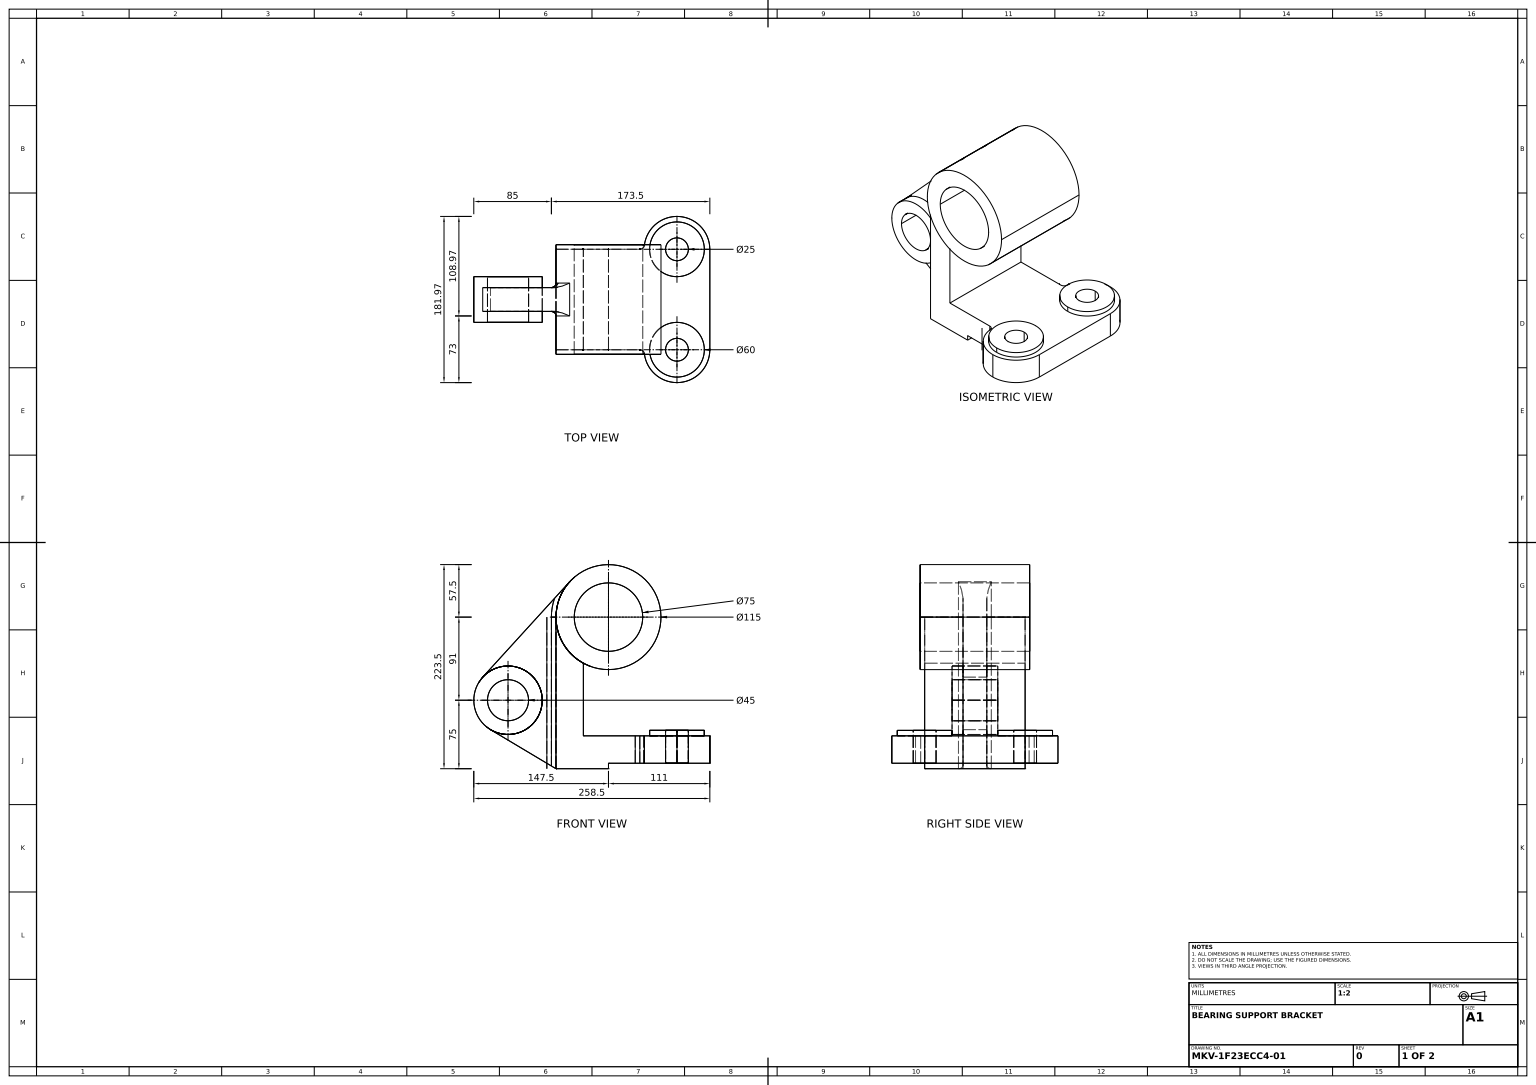
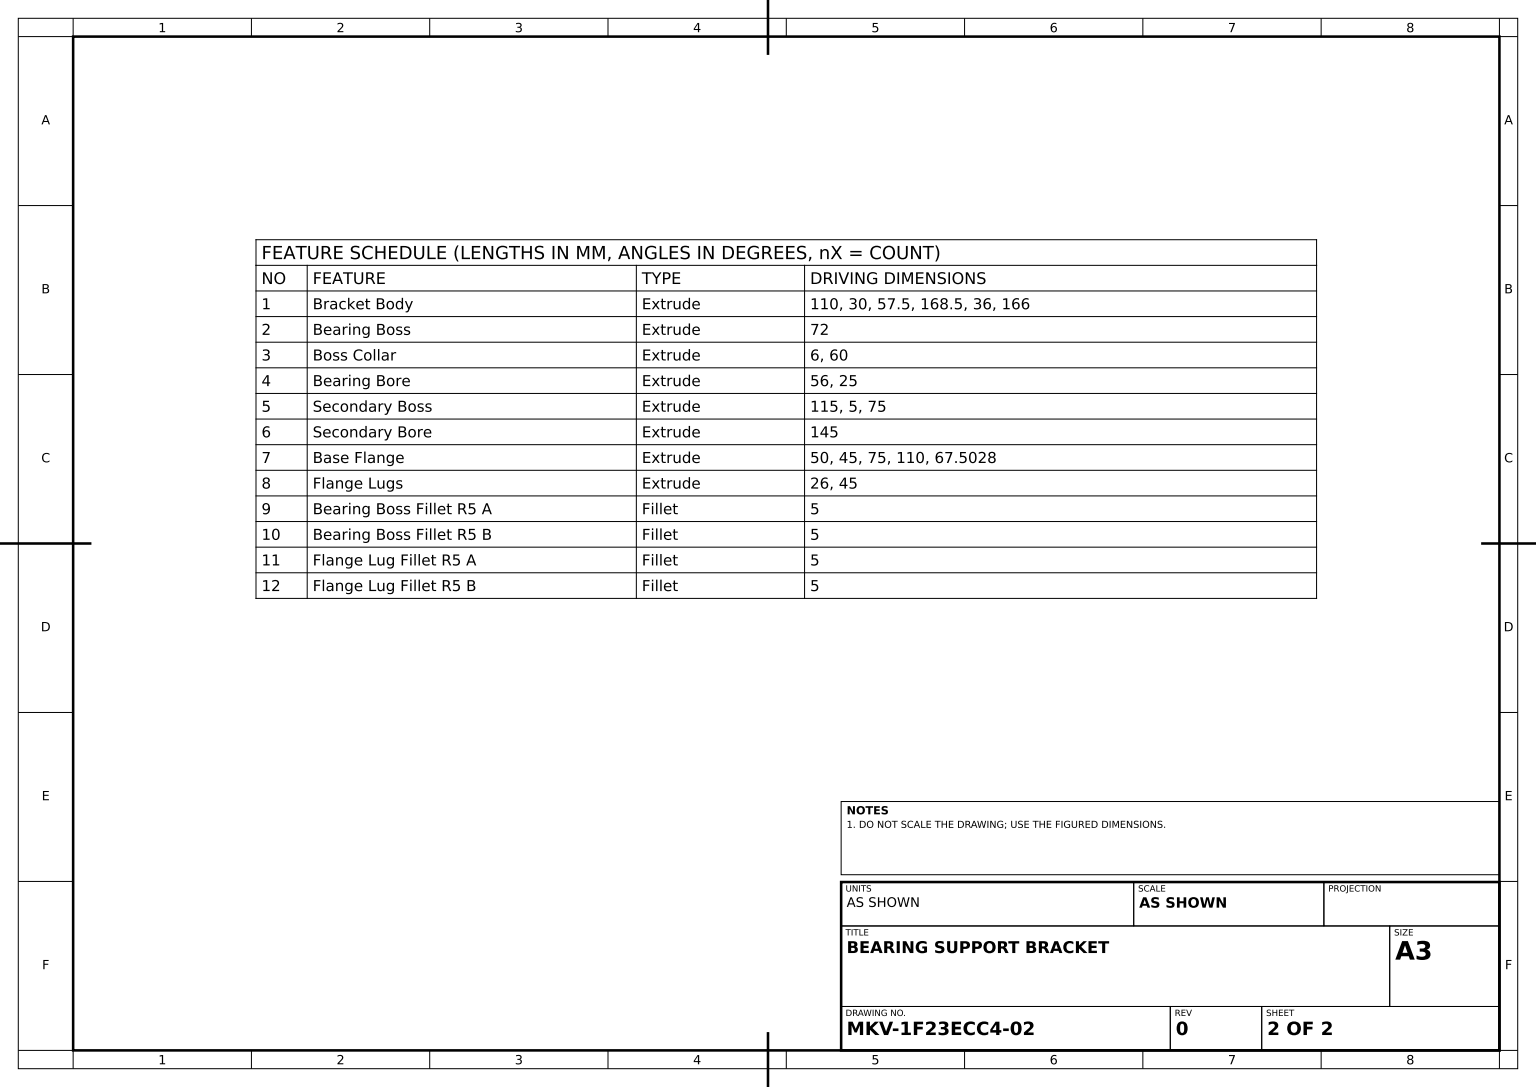
ISO-10303-21;
HEADER;
FILE_DESCRIPTION((''),'2;1');
FILE_NAME('','',(''),(''),'','','');
FILE_SCHEMA(('AUTOMOTIVE_DESIGN'));
ENDSEC;
DATA;
#1=APPLICATION_CONTEXT('');
#2=PRODUCT_CONTEXT('',#1,'mechanical');
#3=PRODUCT('','','',(#2));
#4=PRODUCT_DEFINITION_FORMATION('','',#3);
#5=PRODUCT_DEFINITION_CONTEXT('',#1,'design');
#6=PRODUCT_DEFINITION('','',#4,#5);
#7=PRODUCT_DEFINITION_SHAPE('','',#6);
#8=(LENGTH_UNIT()NAMED_UNIT(*)SI_UNIT(.MILLI.,.METRE.));
#9=(NAMED_UNIT(*)PLANE_ANGLE_UNIT()SI_UNIT($,.RADIAN.));
#10=(NAMED_UNIT(*)SI_UNIT($,.STERADIAN.)SOLID_ANGLE_UNIT());
#11=UNCERTAINTY_MEASURE_WITH_UNIT(LENGTH_MEASURE(1.E-05),#8,'distance_accuracy_value','');
#12=(GEOMETRIC_REPRESENTATION_CONTEXT(3)GLOBAL_UNCERTAINTY_ASSIGNED_CONTEXT((#11))GLOBAL_UNIT_ASSIGNED_CONTEXT((#8,#9,#10))REPRESENTATION_CONTEXT('',''));
#13=CARTESIAN_POINT('',(-75.,75.,-25.));
#14=VERTEX_POINT('',#13);
#15=CARTESIAN_POINT('',(-30.,75.,-25.));
#16=VERTEX_POINT('',#15);
#17=CARTESIAN_POINT('',(-52.5,75.,-25.));
#18=DIRECTION('',(0.,0.,1.));
#19=DIRECTION('',(1.,0.,0.));
#20=AXIS2_PLACEMENT_3D('',#17,#18,#19);
#21=CIRCLE('',#20,22.5);
#22=EDGE_CURVE('',#14,#16,#21,.T.);
#23=ORIENTED_EDGE('',*,*,#22,.T.);
#24=EDGE_CURVE('',#16,#14,#21,.T.);
#25=ORIENTED_EDGE('',*,*,#24,.T.);
#26=EDGE_LOOP('',(#23,#25));
#27=FACE_BOUND('',#26,.T.);
#28=CARTESIAN_POINT('',(-15.,75.,-25.));
#29=VERTEX_POINT('',#28);
#30=CARTESIAN_POINT('',(-90.,75.,-25.));
#31=VERTEX_POINT('',#30);
#32=CIRCLE('',#20,37.5);
#33=EDGE_CURVE('',#29,#31,#32,.T.);
#34=ORIENTED_EDGE('',*,*,#33,.F.);
#35=EDGE_CURVE('',#31,#29,#32,.T.);
#36=ORIENTED_EDGE('',*,*,#35,.F.);
#37=EDGE_LOOP('',(#34,#36));
#38=FACE_OUTER_BOUND('',#37,.T.);
#39=CARTESIAN_POINT('',(0.,0.,-25.));
#40=AXIS2_PLACEMENT_3D('',#39,#18,#19);
#41=PLANE('',#40);
#42=ADVANCED_FACE('',(#27,#38),#41,.F.);
#43=CARTESIAN_POINT('',(30.,36.,55.));
#44=VERTEX_POINT('',#43);
#45=CARTESIAN_POINT('',(30.,115.502475,55.));
#46=VERTEX_POINT('',#45);
#47=DIRECTION('',(0.,1.,0.));
#48=VECTOR('',#47,1000.);
#49=LINE('',#43,#48);
#50=EDGE_CURVE('',#44,#46,#49,.T.);
#51=ORIENTED_EDGE('',*,*,#50,.F.);
#52=CARTESIAN_POINT('',(30.,36.,-55.));
#53=VERTEX_POINT('',#52);
#54=DIRECTION('',(0.,0.,-1.));
#55=VECTOR('',#54,1000.);
#56=LINE('',#43,#55);
#57=EDGE_CURVE('',#44,#53,#56,.T.);
#58=ORIENTED_EDGE('',*,*,#57,.T.);
#59=CARTESIAN_POINT('',(30.,115.502475,-55.));
#60=VERTEX_POINT('',#59);
#61=LINE('',#52,#48);
#62=EDGE_CURVE('',#53,#60,#61,.T.);
#63=ORIENTED_EDGE('',*,*,#62,.T.);
#64=CARTESIAN_POINT('',(30.,115.502475,60.));
#65=LINE('',#64,#55);
#66=EDGE_CURVE('',#46,#60,#65,.T.);
#67=ORIENTED_EDGE('',*,*,#66,.F.);
#68=EDGE_LOOP('',(#51,#58,#63,#67));
#69=FACE_OUTER_BOUND('',#68,.T.);
#70=DIRECTION('',(-1.,0.,0.));
#71=DIRECTION('',(0.,-1.,0.));
#72=AXIS2_PLACEMENT_3D('',#43,#70,#71);
#73=PLANE('',#72);
#74=ADVANCED_FACE('',(#69),#73,.F.);
#75=CARTESIAN_POINT('',(-1.497355,186.629157,13.));
#76=VERTEX_POINT('',#75);
#77=CARTESIAN_POINT('',(-80.215573,100.260582,13.));
#78=VERTEX_POINT('',#77);
#79=DIRECTION('',(-0.673615532,-0.73908194,0.));
#80=VECTOR('',#79,1000.);
#81=LINE('',#77,#80);
#82=EDGE_CURVE('',#76,#78,#81,.T.);
#83=ORIENTED_EDGE('',*,*,#82,.F.);
#84=CARTESIAN_POINT('',(15.002788,204.732893,18.));
#85=VERTEX_POINT('',#84);
#86=CARTESIAN_POINT('',(-0.790057,187.405195,13.));
#87=CARTESIAN_POINT('',(-0.086672,188.176939,13.050128));
#88=CARTESIAN_POINT('',(1.314429,189.714209,13.222969));
#89=CARTESIAN_POINT('',(2.012125,190.479711,13.345952));
#90=CARTESIAN_POINT('',(4.098718,192.769093,13.798084));
#91=CARTESIAN_POINT('',(5.483281,194.288217,14.210374));
#92=CARTESIAN_POINT('',(8.22755,197.299192,15.156454));
#93=CARTESIAN_POINT('',(9.588678,198.792603,15.691176));
#94=CARTESIAN_POINT('',(11.622818,201.024434,16.535584));
#95=CARTESIAN_POINT('',(12.299582,201.766971,16.824242));
#96=CARTESIAN_POINT('',(13.313784,202.87974,17.262515));
#97=CARTESIAN_POINT('',(13.651694,203.250491,17.40949));
#98=CARTESIAN_POINT('',(14.327357,203.991818,17.704321));
#99=CARTESIAN_POINT('',(14.665836,204.363193,17.852495));
#100=B_SPLINE_CURVE_WITH_KNOTS('',3,(#75,#86,#87,#88,#89,#90,#91,#92,#93,#94,#95,#96,#97,#98,#99,#84),.UNSPECIFIED.,.F.,.F.,(4,2,2,2,2,2,2,4),(0.,0.003129059,0.006258119,0.012516238,0.018774357,0.021903416,0.023467946,0.025032475),.UNSPECIFIED.);
#101=EDGE_CURVE('',#76,#85,#100,.T.);
#102=ORIENTED_EDGE('',*,*,#101,.T.);
#103=CARTESIAN_POINT('',(15.002788,204.732893,-18.));
#104=VERTEX_POINT('',#103);
#105=CARTESIAN_POINT('',(15.002788,204.732893,13.));
#106=LINE('',#105,#55);
#107=EDGE_CURVE('',#85,#104,#106,.T.);
#108=ORIENTED_EDGE('',*,*,#107,.T.);
#109=CARTESIAN_POINT('',(-1.497355,186.629157,-13.));
#110=VERTEX_POINT('',#109);
#111=CARTESIAN_POINT('',(13.652305,203.251161,-17.408809));
#112=CARTESIAN_POINT('',(12.300813,201.768322,-16.817032));
#113=CARTESIAN_POINT('',(9.588636,198.792558,-15.69116));
#114=CARTESIAN_POINT('',(8.227513,197.299152,-15.15644));
#115=CARTESIAN_POINT('',(5.483255,194.288189,-14.210366));
#116=CARTESIAN_POINT('',(4.098697,192.76907,-13.798079));
#117=CARTESIAN_POINT('',(2.012112,190.479697,-13.345949));
#118=CARTESIAN_POINT('',(1.314419,189.714197,-13.222967));
#119=CARTESIAN_POINT('',(-0.086678,188.176933,-13.050128));
#120=CARTESIAN_POINT('',(-0.790059,187.405192,-13.));
#121=B_SPLINE_CURVE_WITH_KNOTS('',3,(#103,#111,#112,#113,#114,#115,#116,#117,#118,#119,#120,#109),.UNSPECIFIED.,.F.,.F.,(4,2,2,2,2,4),(-0.000047958,0.006222574,0.012493106,0.018763638,0.021898904,0.025034171),.UNSPECIFIED.);
#122=EDGE_CURVE('',#104,#110,#121,.T.);
#123=ORIENTED_EDGE('',*,*,#122,.T.);
#124=CARTESIAN_POINT('',(-80.215573,100.260582,-13.));
#125=VERTEX_POINT('',#124);
#126=LINE('',#124,#80);
#127=EDGE_CURVE('',#110,#125,#126,.T.);
#128=ORIENTED_EDGE('',*,*,#127,.T.);
#129=LINE('',#77,#55);
#130=EDGE_CURVE('',#78,#125,#129,.T.);
#131=ORIENTED_EDGE('',*,*,#130,.F.);
#132=EDGE_LOOP('',(#83,#102,#108,#123,#128,#131));
#133=FACE_OUTER_BOUND('',#132,.T.);
#134=DIRECTION('',(0.73908194,-0.673615532,0.));
#135=DIRECTION('',(0.673615532,0.73908194,0.));
#136=AXIS2_PLACEMENT_3D('',#77,#134,#135);
#137=PLANE('',#136);
#138=ADVANCED_FACE('',(#133),#137,.F.);
#139=CARTESIAN_POINT('',(-90.,75.,25.));
#140=VERTEX_POINT('',#139);
#141=CARTESIAN_POINT('',(-15.,75.,25.));
#142=VERTEX_POINT('',#141);
#143=CARTESIAN_POINT('',(-52.5,75.,25.));
#144=AXIS2_PLACEMENT_3D('',#143,#18,#19);
#145=CIRCLE('',#144,37.5);
#146=EDGE_CURVE('',#140,#142,#145,.T.);
#147=ORIENTED_EDGE('',*,*,#146,.F.);
#148=CARTESIAN_POINT('',(-90.,75.,13.));
#149=LINE('',#148,#55);
#150=EDGE_CURVE('',#140,#31,#149,.T.);
#151=ORIENTED_EDGE('',*,*,#150,.T.);
#152=ORIENTED_EDGE('',*,*,#35,.T.);
#153=CARTESIAN_POINT('',(-15.,75.,-13.));
#154=VERTEX_POINT('',#153);
#155=CARTESIAN_POINT('',(-15.,75.,13.));
#156=LINE('',#155,#55);
#157=EDGE_CURVE('',#154,#29,#156,.T.);
#158=ORIENTED_EDGE('',*,*,#157,.F.);
#159=CARTESIAN_POINT('',(-71.716935,42.798146,-13.));
#160=VERTEX_POINT('',#159);
#161=CARTESIAN_POINT('',(-52.5,75.,-13.));
#162=AXIS2_PLACEMENT_3D('',#161,#54,#19);
#163=CIRCLE('',#162,37.5);
#164=EDGE_CURVE('',#154,#160,#163,.T.);
#165=ORIENTED_EDGE('',*,*,#164,.T.);
#166=CARTESIAN_POINT('',(-71.716935,42.798146,13.));
#167=VERTEX_POINT('',#166);
#168=LINE('',#166,#55);
#169=EDGE_CURVE('',#167,#160,#168,.T.);
#170=ORIENTED_EDGE('',*,*,#169,.F.);
#171=VERTEX_POINT('',#155);
#172=CARTESIAN_POINT('',(-52.5,75.,13.));
#173=AXIS2_PLACEMENT_3D('',#172,#54,#19);
#174=CIRCLE('',#173,37.5);
#175=EDGE_CURVE('',#171,#167,#174,.T.);
#176=ORIENTED_EDGE('',*,*,#175,.F.);
#177=EDGE_CURVE('',#142,#171,#156,.T.);
#178=ORIENTED_EDGE('',*,*,#177,.F.);
#179=EDGE_LOOP('',(#147,#151,#152,#158,#165,#170,#176,#178));
#180=FACE_OUTER_BOUND('',#179,.T.);
#181=AXIS2_PLACEMENT_3D('',#172,#54,#70);
#182=CYLINDRICAL_SURFACE('',#181,37.5);
#183=ADVANCED_FACE('',(#180),#182,.T.);
#184=CARTESIAN_POINT('',(96.768701,36.,59.390244));
#185=VERTEX_POINT('',#184);
#186=CARTESIAN_POINT('',(96.768701,6.,59.390244));
#187=VERTEX_POINT('',#186);
#188=CARTESIAN_POINT('',(96.768701,-95.823376,59.390244));
#189=VECTOR('',#71,1000.);
#190=LINE('',#188,#189);
#191=EDGE_CURVE('',#185,#187,#190,.T.);
#192=ORIENTED_EDGE('',*,*,#191,.T.);
#193=CARTESIAN_POINT('',(132.5,6.,91.));
#194=VERTEX_POINT('',#193);
#195=CARTESIAN_POINT('',(132.5,6.,55.));
#196=AXIS2_PLACEMENT_3D('',#195,#71,#70);
#197=CIRCLE('',#196,36.);
#198=EDGE_CURVE('',#194,#187,#197,.T.);
#199=ORIENTED_EDGE('',*,*,#198,.F.);
#200=CARTESIAN_POINT('',(132.5,36.,91.));
#201=VERTEX_POINT('',#200);
#202=CARTESIAN_POINT('',(132.5,-95.823376,91.));
#203=LINE('',#202,#48);
#204=EDGE_CURVE('',#194,#201,#203,.T.);
#205=ORIENTED_EDGE('',*,*,#204,.T.);
#206=CARTESIAN_POINT('',(132.5,36.,55.));
#207=AXIS2_PLACEMENT_3D('',#206,#47,#18);
#208=CIRCLE('',#207,36.);
#209=EDGE_CURVE('',#185,#201,#208,.T.);
#210=ORIENTED_EDGE('',*,*,#209,.F.);
#211=EDGE_LOOP('',(#192,#199,#205,#210));
#212=FACE_OUTER_BOUND('',#211,.T.);
#213=CARTESIAN_POINT('',(132.5,-95.823376,55.));
#214=AXIS2_PLACEMENT_3D('',#213,#47,#18);
#215=CYLINDRICAL_SURFACE('',#214,36.);
#216=ADVANCED_FACE('',(#212),#215,.T.);
#217=CARTESIAN_POINT('',(96.768701,6.,-59.390244));
#218=VERTEX_POINT('',#217);
#219=CARTESIAN_POINT('',(96.768701,36.,-59.390244));
#220=VERTEX_POINT('',#219);
#221=CARTESIAN_POINT('',(96.768701,-95.823376,-59.390244));
#222=LINE('',#221,#48);
#223=EDGE_CURVE('',#218,#220,#222,.T.);
#224=ORIENTED_EDGE('',*,*,#223,.T.);
#225=CARTESIAN_POINT('',(168.5,36.,-55.));
#226=VERTEX_POINT('',#225);
#227=CARTESIAN_POINT('',(132.5,36.,-55.));
#228=AXIS2_PLACEMENT_3D('',#227,#47,#18);
#229=CIRCLE('',#228,36.);
#230=EDGE_CURVE('',#226,#220,#229,.T.);
#231=ORIENTED_EDGE('',*,*,#230,.F.);
#232=CARTESIAN_POINT('',(168.5,6.,-55.));
#233=VERTEX_POINT('',#232);
#234=LINE('',#232,#48);
#235=EDGE_CURVE('',#233,#226,#234,.T.);
#236=ORIENTED_EDGE('',*,*,#235,.F.);
#237=CARTESIAN_POINT('',(132.5,6.,-55.));
#238=AXIS2_PLACEMENT_3D('',#237,#71,#70);
#239=CIRCLE('',#238,36.);
#240=EDGE_CURVE('',#218,#233,#239,.T.);
#241=ORIENTED_EDGE('',*,*,#240,.F.);
#242=EDGE_LOOP('',(#224,#231,#236,#241));
#243=FACE_OUTER_BOUND('',#242,.T.);
#244=CARTESIAN_POINT('',(132.5,-95.823376,-55.));
#245=AXIS2_PLACEMENT_3D('',#244,#47,#18);
#246=CYLINDRICAL_SURFACE('',#245,36.);
#247=ADVANCED_FACE('',(#243),#246,.T.);
#248=CARTESIAN_POINT('',(95.,166.,60.));
#249=VERTEX_POINT('',#248);
#250=CARTESIAN_POINT('',(95.,166.,-60.));
#251=VERTEX_POINT('',#250);
#252=LINE('',#248,#55);
#253=EDGE_CURVE('',#249,#251,#252,.T.);
#254=ORIENTED_EDGE('',*,*,#253,.T.);
#255=CARTESIAN_POINT('',(20.,166.,-60.));
#256=VERTEX_POINT('',#255);
#257=CARTESIAN_POINT('',(57.5,166.,-60.));
#258=AXIS2_PLACEMENT_3D('',#257,#18,#19);
#259=CIRCLE('',#258,37.5);
#260=EDGE_CURVE('',#256,#251,#259,.T.);
#261=ORIENTED_EDGE('',*,*,#260,.F.);
#262=CARTESIAN_POINT('',(20.,166.,60.));
#263=VERTEX_POINT('',#262);
#264=LINE('',#262,#55);
#265=EDGE_CURVE('',#263,#256,#264,.T.);
#266=ORIENTED_EDGE('',*,*,#265,.F.);
#267=CARTESIAN_POINT('',(57.5,166.,60.));
#268=AXIS2_PLACEMENT_3D('',#267,#18,#19);
#269=CIRCLE('',#268,37.5);
#270=EDGE_CURVE('',#263,#249,#269,.T.);
#271=ORIENTED_EDGE('',*,*,#270,.T.);
#272=EDGE_LOOP('',(#254,#261,#266,#271));
#273=FACE_OUTER_BOUND('',#272,.T.);
#274=AXIS2_PLACEMENT_3D('',#267,#54,#70);
#275=CYLINDRICAL_SURFACE('',#274,37.5);
#276=ADVANCED_FACE('',(#273),#275,.F.);
#277=CARTESIAN_POINT('',(-5.,166.,-13.));
#278=VERTEX_POINT('',#277);
#279=CARTESIAN_POINT('',(57.5,166.,-13.));
#280=AXIS2_PLACEMENT_3D('',#279,#18,#19);
#281=CIRCLE('',#280,62.5);
#282=EDGE_CURVE('',#110,#278,#281,.T.);
#283=ORIENTED_EDGE('',*,*,#282,.T.);
#284=CARTESIAN_POINT('',(-5.,2.983824,-13.));
#285=VERTEX_POINT('',#284);
#286=CARTESIAN_POINT('',(-5.,0.,-13.));
#287=LINE('',#286,#189);
#288=EDGE_CURVE('',#278,#285,#287,.T.);
#289=ORIENTED_EDGE('',*,*,#288,.T.);
#290=CARTESIAN_POINT('',(0.,0.,-13.));
#291=DIRECTION('',(0.858716115,-0.512451592,0.));
#292=VECTOR('',#291,1000.);
#293=LINE('',#290,#292);
#294=EDGE_CURVE('',#160,#285,#293,.T.);
#295=ORIENTED_EDGE('',*,*,#294,.F.);
#296=ORIENTED_EDGE('',*,*,#164,.F.);
#297=EDGE_CURVE('',#125,#154,#163,.T.);
#298=ORIENTED_EDGE('',*,*,#297,.F.);
#299=ORIENTED_EDGE('',*,*,#127,.F.);
#300=EDGE_LOOP('',(#283,#289,#295,#296,#298,#299));
#301=FACE_OUTER_BOUND('',#300,.T.);
#302=AXIS2_PLACEMENT_3D('',#161,#18,#19);
#303=PLANE('',#302);
#304=ADVANCED_FACE('',(#301),#303,.F.);
#305=CARTESIAN_POINT('',(168.5,6.,55.));
#306=VERTEX_POINT('',#305);
#307=CARTESIAN_POINT('',(168.5,36.,55.));
#308=VERTEX_POINT('',#307);
#309=LINE('',#305,#48);
#310=EDGE_CURVE('',#306,#308,#309,.T.);
#311=ORIENTED_EDGE('',*,*,#310,.T.);
#312=EDGE_CURVE('',#201,#308,#208,.T.);
#313=ORIENTED_EDGE('',*,*,#312,.F.);
#314=ORIENTED_EDGE('',*,*,#204,.F.);
#315=EDGE_CURVE('',#306,#194,#197,.T.);
#316=ORIENTED_EDGE('',*,*,#315,.F.);
#317=EDGE_LOOP('',(#311,#313,#314,#316));
#318=FACE_OUTER_BOUND('',#317,.T.);
#319=ADVANCED_FACE('',(#318),#215,.T.);
#320=EDGE_CURVE('',#251,#256,#259,.T.);
#321=ORIENTED_EDGE('',*,*,#320,.F.);
#322=ORIENTED_EDGE('',*,*,#253,.F.);
#323=EDGE_CURVE('',#249,#263,#269,.T.);
#324=ORIENTED_EDGE('',*,*,#323,.T.);
#325=ORIENTED_EDGE('',*,*,#265,.T.);
#326=EDGE_LOOP('',(#321,#322,#324,#325));
#327=FACE_OUTER_BOUND('',#326,.T.);
#328=ADVANCED_FACE('',(#327),#275,.F.);
#329=CARTESIAN_POINT('',(0.,0.,-55.));
#330=VERTEX_POINT('',#329);
#331=CARTESIAN_POINT('',(57.5,0.,-55.));
#332=VERTEX_POINT('',#331);
#333=VECTOR('',#19,1000.);
#334=LINE('',#329,#333);
#335=EDGE_CURVE('',#330,#332,#334,.T.);
#336=ORIENTED_EDGE('',*,*,#335,.F.);
#337=CARTESIAN_POINT('',(0.,166.,-55.));
#338=VERTEX_POINT('',#337);
#339=LINE('',#337,#189);
#340=EDGE_CURVE('',#338,#330,#339,.T.);
#341=ORIENTED_EDGE('',*,*,#340,.F.);
#342=CARTESIAN_POINT('',(57.5,166.,-55.));
#343=AXIS2_PLACEMENT_3D('',#342,#54,#19);
#344=CIRCLE('',#343,57.5);
#345=EDGE_CURVE('',#60,#338,#344,.T.);
#346=ORIENTED_EDGE('',*,*,#345,.F.);
#347=ORIENTED_EDGE('',*,*,#62,.F.);
#348=CARTESIAN_POINT('',(91.80602,36.,-55.));
#349=VERTEX_POINT('',#348);
#350=VECTOR('',#70,1000.);
#351=LINE('',#225,#350);
#352=EDGE_CURVE('',#349,#53,#351,.T.);
#353=ORIENTED_EDGE('',*,*,#352,.F.);
#354=CARTESIAN_POINT('',(91.80602,6.,-55.));
#355=VERTEX_POINT('',#354);
#356=CARTESIAN_POINT('',(91.80602,0.,-55.));
#357=LINE('',#356,#189);
#358=EDGE_CURVE('',#349,#355,#357,.T.);
#359=ORIENTED_EDGE('',*,*,#358,.T.);
#360=CARTESIAN_POINT('',(57.5,6.,-55.));
#361=VERTEX_POINT('',#360);
#362=LINE('',#360,#333);
#363=EDGE_CURVE('',#361,#355,#362,.T.);
#364=ORIENTED_EDGE('',*,*,#363,.F.);
#365=LINE('',#331,#48);
#366=EDGE_CURVE('',#332,#361,#365,.T.);
#367=ORIENTED_EDGE('',*,*,#366,.F.);
#368=EDGE_LOOP('',(#336,#341,#346,#347,#353,#359,#364,#367));
#369=FACE_OUTER_BOUND('',#368,.T.);
#370=AXIS2_PLACEMENT_3D('',#329,#18,#19);
#371=PLANE('',#370);
#372=ADVANCED_FACE('',(#369),#371,.F.);
#373=EDGE_CURVE('',#142,#140,#145,.T.);
#374=ORIENTED_EDGE('',*,*,#373,.T.);
#375=ORIENTED_EDGE('',*,*,#146,.T.);
#376=EDGE_LOOP('',(#374,#375));
#377=FACE_OUTER_BOUND('',#376,.T.);
#378=CARTESIAN_POINT('',(-30.,75.,25.));
#379=VERTEX_POINT('',#378);
#380=CARTESIAN_POINT('',(-75.,75.,25.));
#381=VERTEX_POINT('',#380);
#382=CIRCLE('',#144,22.5);
#383=EDGE_CURVE('',#379,#381,#382,.T.);
#384=ORIENTED_EDGE('',*,*,#383,.F.);
#385=EDGE_CURVE('',#381,#379,#382,.T.);
#386=ORIENTED_EDGE('',*,*,#385,.F.);
#387=EDGE_LOOP('',(#384,#386));
#388=FACE_BOUND('',#387,.T.);
#389=CARTESIAN_POINT('',(0.,0.,25.));
#390=AXIS2_PLACEMENT_3D('',#389,#18,#19);
#391=PLANE('',#390);
#392=ADVANCED_FACE('',(#377,#388),#391,.T.);
#393=ORIENTED_EDGE('',*,*,#270,.F.);
#394=ORIENTED_EDGE('',*,*,#323,.F.);
#395=EDGE_LOOP('',(#393,#394));
#396=FACE_BOUND('',#395,.T.);
#397=CARTESIAN_POINT('',(0.,166.,60.));
#398=VERTEX_POINT('',#397);
#399=CARTESIAN_POINT('',(115.,166.,60.));
#400=VERTEX_POINT('',#399);
#401=CIRCLE('',#268,57.5);
#402=EDGE_CURVE('',#398,#400,#401,.T.);
#403=ORIENTED_EDGE('',*,*,#402,.T.);
#404=EDGE_CURVE('',#400,#398,#401,.T.);
#405=ORIENTED_EDGE('',*,*,#404,.T.);
#406=EDGE_LOOP('',(#403,#405));
#407=FACE_OUTER_BOUND('',#406,.T.);
#408=PLANE('',#268);
#409=ADVANCED_FACE('',(#396,#407),#408,.T.);
#410=CARTESIAN_POINT('',(-5.,166.,13.));
#411=VERTEX_POINT('',#410);
#412=CARTESIAN_POINT('',(57.5,166.,13.));
#413=AXIS2_PLACEMENT_3D('',#412,#54,#19);
#414=CIRCLE('',#413,62.5);
#415=EDGE_CURVE('',#411,#76,#414,.T.);
#416=ORIENTED_EDGE('',*,*,#415,.F.);
#417=CARTESIAN_POINT('',(0.,166.,18.));
#418=VERTEX_POINT('',#417);
#419=CARTESIAN_POINT('',(-5.,166.,18.));
#420=AXIS2_PLACEMENT_3D('',#419,#71,#54);
#421=CIRCLE('',#420,5.);
#422=EDGE_CURVE('',#411,#418,#421,.T.);
#423=ORIENTED_EDGE('',*,*,#422,.T.);
#424=CARTESIAN_POINT('',(57.5,166.,18.));
#425=AXIS2_PLACEMENT_3D('',#424,#18,#19);
#426=CIRCLE('',#425,57.5);
#427=EDGE_CURVE('',#85,#418,#426,.T.);
#428=ORIENTED_EDGE('',*,*,#427,.F.);
#429=ORIENTED_EDGE('',*,*,#101,.F.);
#430=EDGE_LOOP('',(#416,#423,#428,#429));
#431=FACE_OUTER_BOUND('',#430,.T.);
#432=TOROIDAL_SURFACE('',#425,62.5,5.);
#433=ADVANCED_FACE('',(#431),#432,.F.);
#434=ORIENTED_EDGE('',*,*,#288,.F.);
#435=CARTESIAN_POINT('',(0.,166.,-18.));
#436=VERTEX_POINT('',#435);
#437=CARTESIAN_POINT('',(-5.,166.,-18.));
#438=AXIS2_PLACEMENT_3D('',#437,#71,#54);
#439=CIRCLE('',#438,5.);
#440=EDGE_CURVE('',#436,#278,#439,.T.);
#441=ORIENTED_EDGE('',*,*,#440,.F.);
#442=CARTESIAN_POINT('',(0.,0.,-18.));
#443=VERTEX_POINT('',#442);
#444=LINE('',#435,#48);
#445=EDGE_CURVE('',#443,#436,#444,.T.);
#446=ORIENTED_EDGE('',*,*,#445,.F.);
#447=CARTESIAN_POINT('',(-2.071068,1.23594,-13.));
#448=CARTESIAN_POINT('',(0.,0.,-15.071068));
#449=(BOUNDED_CURVE()B_SPLINE_CURVE(3,(#284,#447,#448,#442),.UNSPECIFIED.,.F.,.T.)B_SPLINE_CURVE_WITH_KNOTS((4,4),(4.71238898,6.283185307),.UNSPECIFIED.)CURVE()GEOMETRIC_REPRESENTATION_ITEM()RATIONAL_B_SPLINE_CURVE((1.,0.804737854,0.804737854,1.))REPRESENTATION_ITEM(''));
#450=EDGE_CURVE('',#285,#443,#449,.T.);
#451=ORIENTED_EDGE('',*,*,#450,.F.);
#452=EDGE_LOOP('',(#434,#441,#446,#451));
#453=FACE_OUTER_BOUND('',#452,.T.);
#454=AXIS2_PLACEMENT_3D('',#437,#71,#19);
#455=CYLINDRICAL_SURFACE('',#454,5.);
#456=ADVANCED_FACE('',(#453),#455,.F.);
#457=ORIENTED_EDGE('',*,*,#358,.F.);
#458=CARTESIAN_POINT('',(91.80602,36.,-60.));
#459=AXIS2_PLACEMENT_3D('',#458,#71,#54);
#460=CIRCLE('',#459,5.);
#461=EDGE_CURVE('',#220,#349,#460,.T.);
#462=ORIENTED_EDGE('',*,*,#461,.F.);
#463=ORIENTED_EDGE('',*,*,#223,.F.);
#464=CARTESIAN_POINT('',(91.80602,6.,-60.));
#465=AXIS2_PLACEMENT_3D('',#464,#47,#70);
#466=CIRCLE('',#465,5.);
#467=EDGE_CURVE('',#355,#218,#466,.T.);
#468=ORIENTED_EDGE('',*,*,#467,.F.);
#469=EDGE_LOOP('',(#457,#462,#463,#468));
#470=FACE_OUTER_BOUND('',#469,.T.);
#471=CARTESIAN_POINT('',(91.80602,-95.823376,-60.));
#472=AXIS2_PLACEMENT_3D('',#471,#47,#18);
#473=CYLINDRICAL_SURFACE('',#472,5.);
#474=ADVANCED_FACE('',(#470),#473,.F.);
#475=CARTESIAN_POINT('',(132.5,42.,-42.5));
#476=VERTEX_POINT('',#475);
#477=CARTESIAN_POINT('',(132.5,42.,-67.5));
#478=VERTEX_POINT('',#477);
#479=CARTESIAN_POINT('',(132.5,42.,-55.));
#480=AXIS2_PLACEMENT_3D('',#479,#47,#18);
#481=CIRCLE('',#480,12.5);
#482=EDGE_CURVE('',#476,#478,#481,.T.);
#483=ORIENTED_EDGE('',*,*,#482,.T.);
#484=CARTESIAN_POINT('',(132.5,6.,-67.5));
#485=VERTEX_POINT('',#484);
#486=CARTESIAN_POINT('',(132.5,-14.,-67.5));
#487=LINE('',#486,#48);
#488=EDGE_CURVE('',#485,#478,#487,.T.);
#489=ORIENTED_EDGE('',*,*,#488,.F.);
#490=CARTESIAN_POINT('',(132.5,6.,-42.5));
#491=VERTEX_POINT('',#490);
#492=AXIS2_PLACEMENT_3D('',#237,#47,#70);
#493=CIRCLE('',#492,12.5);
#494=EDGE_CURVE('',#491,#485,#493,.T.);
#495=ORIENTED_EDGE('',*,*,#494,.F.);
#496=CARTESIAN_POINT('',(132.5,-14.,-42.5));
#497=LINE('',#496,#48);
#498=EDGE_CURVE('',#491,#476,#497,.T.);
#499=ORIENTED_EDGE('',*,*,#498,.T.);
#500=EDGE_LOOP('',(#483,#489,#495,#499));
#501=FACE_OUTER_BOUND('',#500,.T.);
#502=CARTESIAN_POINT('',(132.5,-14.,-55.));
#503=AXIS2_PLACEMENT_3D('',#502,#47,#18);
#504=CYLINDRICAL_SURFACE('',#503,12.5);
#505=ADVANCED_FACE('',(#501),#504,.F.);
#506=ORIENTED_EDGE('',*,*,#450,.T.);
#507=CARTESIAN_POINT('',(0.,0.,18.));
#508=VERTEX_POINT('',#507);
#509=CARTESIAN_POINT('',(0.,0.,13.));
#510=LINE('',#509,#55);
#511=EDGE_CURVE('',#508,#443,#510,.T.);
#512=ORIENTED_EDGE('',*,*,#511,.F.);
#513=CARTESIAN_POINT('',(-5.,2.983824,13.));
#514=VERTEX_POINT('',#513);
#515=CARTESIAN_POINT('',(0.,0.,15.071068));
#516=CARTESIAN_POINT('',(-2.071068,1.23594,13.));
#517=(BOUNDED_CURVE()B_SPLINE_CURVE(3,(#507,#515,#516,#513),.UNSPECIFIED.,.F.,.T.)B_SPLINE_CURVE_WITH_KNOTS((4,4),(3.141592654,4.71238898),.UNSPECIFIED.)CURVE()GEOMETRIC_REPRESENTATION_ITEM()RATIONAL_B_SPLINE_CURVE((1.,0.804737854,0.804737854,1.))REPRESENTATION_ITEM(''));
#518=EDGE_CURVE('',#508,#514,#517,.T.);
#519=ORIENTED_EDGE('',*,*,#518,.T.);
#520=LINE('',#509,#292);
#521=EDGE_CURVE('',#167,#514,#520,.T.);
#522=ORIENTED_EDGE('',*,*,#521,.F.);
#523=ORIENTED_EDGE('',*,*,#169,.T.);
#524=ORIENTED_EDGE('',*,*,#294,.T.);
#525=EDGE_LOOP('',(#506,#512,#519,#522,#523,#524));
#526=FACE_OUTER_BOUND('',#525,.T.);
#527=DIRECTION('',(0.512451592,0.858716115,0.));
#528=DIRECTION('',(-0.858716115,0.512451592,0.));
#529=AXIS2_PLACEMENT_3D('',#509,#527,#528);
#530=PLANE('',#529);
#531=ADVANCED_FACE('',(#526),#530,.F.);
#532=ORIENTED_EDGE('',*,*,#440,.T.);
#533=ORIENTED_EDGE('',*,*,#282,.F.);
#534=ORIENTED_EDGE('',*,*,#122,.F.);
#535=CARTESIAN_POINT('',(57.5,166.,-18.));
#536=AXIS2_PLACEMENT_3D('',#535,#54,#19);
#537=CIRCLE('',#536,57.5);
#538=EDGE_CURVE('',#436,#104,#537,.T.);
#539=ORIENTED_EDGE('',*,*,#538,.F.);
#540=EDGE_LOOP('',(#532,#533,#534,#539));
#541=FACE_OUTER_BOUND('',#540,.T.);
#542=AXIS2_PLACEMENT_3D('',#535,#18,#19);
#543=TOROIDAL_SURFACE('',#542,62.5,5.);
#544=ADVANCED_FACE('',(#541),#543,.F.);
#545=CARTESIAN_POINT('',(132.5,42.,-25.));
#546=VERTEX_POINT('',#545);
#547=CARTESIAN_POINT('',(132.5,42.,-85.));
#548=VERTEX_POINT('',#547);
#549=CIRCLE('',#480,30.);
#550=EDGE_CURVE('',#546,#548,#549,.T.);
#551=ORIENTED_EDGE('',*,*,#550,.T.);
#552=EDGE_CURVE('',#548,#546,#549,.T.);
#553=ORIENTED_EDGE('',*,*,#552,.T.);
#554=EDGE_LOOP('',(#551,#553));
#555=FACE_OUTER_BOUND('',#554,.T.);
#556=EDGE_CURVE('',#478,#476,#481,.T.);
#557=ORIENTED_EDGE('',*,*,#556,.F.);
#558=ORIENTED_EDGE('',*,*,#482,.F.);
#559=EDGE_LOOP('',(#557,#558));
#560=FACE_BOUND('',#559,.T.);
#561=PLANE('',#480);
#562=ADVANCED_FACE('',(#555,#560),#561,.T.);
#563=CARTESIAN_POINT('',(132.5,6.,67.5));
#564=VERTEX_POINT('',#563);
#565=CARTESIAN_POINT('',(132.5,6.,42.5));
#566=VERTEX_POINT('',#565);
#567=AXIS2_PLACEMENT_3D('',#195,#47,#70);
#568=CIRCLE('',#567,12.5);
#569=EDGE_CURVE('',#564,#566,#568,.T.);
#570=ORIENTED_EDGE('',*,*,#569,.F.);
#571=CARTESIAN_POINT('',(132.5,42.,67.5));
#572=VERTEX_POINT('',#571);
#573=CARTESIAN_POINT('',(132.5,-14.,67.5));
#574=LINE('',#573,#48);
#575=EDGE_CURVE('',#564,#572,#574,.T.);
#576=ORIENTED_EDGE('',*,*,#575,.T.);
#577=CARTESIAN_POINT('',(132.5,42.,42.5));
#578=VERTEX_POINT('',#577);
#579=CARTESIAN_POINT('',(132.5,42.,55.));
#580=AXIS2_PLACEMENT_3D('',#579,#47,#18);
#581=CIRCLE('',#580,12.5);
#582=EDGE_CURVE('',#572,#578,#581,.T.);
#583=ORIENTED_EDGE('',*,*,#582,.T.);
#584=CARTESIAN_POINT('',(132.5,-14.,42.5));
#585=LINE('',#584,#48);
#586=EDGE_CURVE('',#566,#578,#585,.T.);
#587=ORIENTED_EDGE('',*,*,#586,.F.);
#588=EDGE_LOOP('',(#570,#576,#583,#587));
#589=FACE_OUTER_BOUND('',#588,.T.);
#590=CARTESIAN_POINT('',(132.5,-14.,55.));
#591=AXIS2_PLACEMENT_3D('',#590,#47,#18);
#592=CYLINDRICAL_SURFACE('',#591,12.5);
#593=ADVANCED_FACE('',(#589),#592,.F.);
#594=CARTESIAN_POINT('',(132.5,42.,25.));
#595=VERTEX_POINT('',#594);
#596=CARTESIAN_POINT('',(132.5,36.,25.));
#597=VERTEX_POINT('',#596);
#598=LINE('',#594,#189);
#599=EDGE_CURVE('',#595,#597,#598,.T.);
#600=ORIENTED_EDGE('',*,*,#599,.F.);
#601=CARTESIAN_POINT('',(132.5,42.,85.));
#602=VERTEX_POINT('',#601);
#603=CIRCLE('',#580,30.);
#604=EDGE_CURVE('',#602,#595,#603,.T.);
#605=ORIENTED_EDGE('',*,*,#604,.F.);
#606=CARTESIAN_POINT('',(132.5,36.,85.));
#607=VERTEX_POINT('',#606);
#608=LINE('',#601,#189);
#609=EDGE_CURVE('',#602,#607,#608,.T.);
#610=ORIENTED_EDGE('',*,*,#609,.T.);
#611=AXIS2_PLACEMENT_3D('',#206,#47,#54);
#612=CIRCLE('',#611,30.);
#613=EDGE_CURVE('',#607,#597,#612,.T.);
#614=ORIENTED_EDGE('',*,*,#613,.T.);
#615=EDGE_LOOP('',(#600,#605,#610,#614));
#616=FACE_OUTER_BOUND('',#615,.T.);
#617=AXIS2_PLACEMENT_3D('',#579,#71,#54);
#618=CYLINDRICAL_SURFACE('',#617,30.);
#619=ADVANCED_FACE('',(#616),#618,.T.);
#620=ORIENTED_EDGE('',*,*,#569,.T.);
#621=EDGE_CURVE('',#566,#564,#568,.T.);
#622=ORIENTED_EDGE('',*,*,#621,.T.);
#623=EDGE_LOOP('',(#620,#622));
#624=FACE_BOUND('',#623,.T.);
#625=ORIENTED_EDGE('',*,*,#494,.T.);
#626=EDGE_CURVE('',#485,#491,#493,.T.);
#627=ORIENTED_EDGE('',*,*,#626,.T.);
#628=EDGE_LOOP('',(#625,#627));
#629=FACE_BOUND('',#628,.T.);
#630=ORIENTED_EDGE('',*,*,#363,.T.);
#631=ORIENTED_EDGE('',*,*,#467,.T.);
#632=ORIENTED_EDGE('',*,*,#240,.T.);
#633=LINE('',#305,#55);
#634=EDGE_CURVE('',#306,#233,#633,.T.);
#635=ORIENTED_EDGE('',*,*,#634,.F.);
#636=ORIENTED_EDGE('',*,*,#315,.T.);
#637=ORIENTED_EDGE('',*,*,#198,.T.);
#638=CARTESIAN_POINT('',(91.80602,6.,55.));
#639=VERTEX_POINT('',#638);
#640=CARTESIAN_POINT('',(91.80602,6.,60.));
#641=AXIS2_PLACEMENT_3D('',#640,#47,#70);
#642=CIRCLE('',#641,5.);
#643=EDGE_CURVE('',#187,#639,#642,.T.);
#644=ORIENTED_EDGE('',*,*,#643,.T.);
#645=CARTESIAN_POINT('',(57.5,6.,55.));
#646=VERTEX_POINT('',#645);
#647=LINE('',#645,#333);
#648=EDGE_CURVE('',#646,#639,#647,.T.);
#649=ORIENTED_EDGE('',*,*,#648,.F.);
#650=LINE('',#645,#55);
#651=EDGE_CURVE('',#646,#361,#650,.T.);
#652=ORIENTED_EDGE('',*,*,#651,.T.);
#653=EDGE_LOOP('',(#630,#631,#632,#635,#636,#637,#644,#649,#652));
#654=FACE_OUTER_BOUND('',#653,.T.);
#655=AXIS2_PLACEMENT_3D('',#645,#47,#70);
#656=PLANE('',#655);
#657=ADVANCED_FACE('',(#624,#629,#654),#656,.F.);
#658=CARTESIAN_POINT('',(-75.,75.,13.));
#659=LINE('',#658,#55);
#660=EDGE_CURVE('',#381,#14,#659,.T.);
#661=ORIENTED_EDGE('',*,*,#660,.F.);
#662=ORIENTED_EDGE('',*,*,#385,.T.);
#663=CARTESIAN_POINT('',(-30.,75.,13.));
#664=LINE('',#663,#55);
#665=EDGE_CURVE('',#379,#16,#664,.T.);
#666=ORIENTED_EDGE('',*,*,#665,.T.);
#667=ORIENTED_EDGE('',*,*,#22,.F.);
#668=EDGE_LOOP('',(#661,#662,#666,#667));
#669=FACE_OUTER_BOUND('',#668,.T.);
#670=CYLINDRICAL_SURFACE('',#181,22.5);
#671=ADVANCED_FACE('',(#669),#670,.F.);
#672=LINE('',#307,#55);
#673=EDGE_CURVE('',#308,#226,#672,.T.);
#674=ORIENTED_EDGE('',*,*,#673,.T.);
#675=ORIENTED_EDGE('',*,*,#230,.T.);
#676=ORIENTED_EDGE('',*,*,#461,.T.);
#677=ORIENTED_EDGE('',*,*,#352,.T.);
#678=ORIENTED_EDGE('',*,*,#57,.F.);
#679=CARTESIAN_POINT('',(91.80602,36.,55.));
#680=VERTEX_POINT('',#679);
#681=LINE('',#307,#350);
#682=EDGE_CURVE('',#680,#44,#681,.T.);
#683=ORIENTED_EDGE('',*,*,#682,.F.);
#684=CARTESIAN_POINT('',(91.80602,36.,60.));
#685=AXIS2_PLACEMENT_3D('',#684,#71,#54);
#686=CIRCLE('',#685,5.);
#687=EDGE_CURVE('',#680,#185,#686,.T.);
#688=ORIENTED_EDGE('',*,*,#687,.T.);
#689=ORIENTED_EDGE('',*,*,#209,.T.);
#690=ORIENTED_EDGE('',*,*,#312,.T.);
#691=EDGE_LOOP('',(#674,#675,#676,#677,#678,#683,#688,#689,#690));
#692=FACE_OUTER_BOUND('',#691,.T.);
#693=CARTESIAN_POINT('',(132.5,36.,-85.));
#694=VERTEX_POINT('',#693);
#695=CARTESIAN_POINT('',(132.5,36.,-25.));
#696=VERTEX_POINT('',#695);
#697=AXIS2_PLACEMENT_3D('',#227,#47,#54);
#698=CIRCLE('',#697,30.);
#699=EDGE_CURVE('',#694,#696,#698,.T.);
#700=ORIENTED_EDGE('',*,*,#699,.F.);
#701=EDGE_CURVE('',#696,#694,#698,.T.);
#702=ORIENTED_EDGE('',*,*,#701,.F.);
#703=EDGE_LOOP('',(#700,#702));
#704=FACE_BOUND('',#703,.T.);
#705=EDGE_CURVE('',#597,#607,#612,.T.);
#706=ORIENTED_EDGE('',*,*,#705,.F.);
#707=ORIENTED_EDGE('',*,*,#613,.F.);
#708=EDGE_LOOP('',(#706,#707));
#709=FACE_BOUND('',#708,.T.);
#710=AXIS2_PLACEMENT_3D('',#307,#71,#54);
#711=PLANE('',#710);
#712=ADVANCED_FACE('',(#692,#704,#709),#711,.F.);
#713=ORIENTED_EDGE('',*,*,#498,.F.);
#714=ORIENTED_EDGE('',*,*,#626,.F.);
#715=ORIENTED_EDGE('',*,*,#488,.T.);
#716=ORIENTED_EDGE('',*,*,#556,.T.);
#717=EDGE_LOOP('',(#713,#714,#715,#716));
#718=FACE_OUTER_BOUND('',#717,.T.);
#719=ADVANCED_FACE('',(#718),#504,.F.);
#720=CARTESIAN_POINT('',(-5.,75.,13.));
#721=LINE('',#720,#48);
#722=EDGE_CURVE('',#514,#411,#721,.T.);
#723=ORIENTED_EDGE('',*,*,#722,.F.);
#724=ORIENTED_EDGE('',*,*,#518,.F.);
#725=LINE('',#417,#189);
#726=EDGE_CURVE('',#418,#508,#725,.T.);
#727=ORIENTED_EDGE('',*,*,#726,.F.);
#728=ORIENTED_EDGE('',*,*,#422,.F.);
#729=EDGE_LOOP('',(#723,#724,#727,#728));
#730=FACE_OUTER_BOUND('',#729,.T.);
#731=CARTESIAN_POINT('',(-5.,75.,18.));
#732=AXIS2_PLACEMENT_3D('',#731,#47,#70);
#733=CYLINDRICAL_SURFACE('',#732,5.);
#734=ADVANCED_FACE('',(#730),#733,.F.);
#735=ORIENTED_EDGE('',*,*,#705,.T.);
#736=ORIENTED_EDGE('',*,*,#609,.F.);
#737=EDGE_CURVE('',#595,#602,#603,.T.);
#738=ORIENTED_EDGE('',*,*,#737,.F.);
#739=ORIENTED_EDGE('',*,*,#599,.T.);
#740=EDGE_LOOP('',(#735,#736,#738,#739));
#741=FACE_OUTER_BOUND('',#740,.T.);
#742=ADVANCED_FACE('',(#741),#618,.T.);
#743=CARTESIAN_POINT('',(0.,0.,55.));
#744=VERTEX_POINT('',#743);
#745=LINE('',#743,#55);
#746=EDGE_CURVE('',#744,#508,#745,.T.);
#747=ORIENTED_EDGE('',*,*,#746,.T.);
#748=ORIENTED_EDGE('',*,*,#511,.T.);
#749=EDGE_CURVE('',#443,#330,#745,.T.);
#750=ORIENTED_EDGE('',*,*,#749,.T.);
#751=ORIENTED_EDGE('',*,*,#335,.T.);
#752=CARTESIAN_POINT('',(57.5,0.,55.));
#753=VERTEX_POINT('',#752);
#754=LINE('',#752,#55);
#755=EDGE_CURVE('',#753,#332,#754,.T.);
#756=ORIENTED_EDGE('',*,*,#755,.F.);
#757=LINE('',#743,#333);
#758=EDGE_CURVE('',#744,#753,#757,.T.);
#759=ORIENTED_EDGE('',*,*,#758,.F.);
#760=EDGE_LOOP('',(#747,#748,#750,#751,#756,#759));
#761=FACE_OUTER_BOUND('',#760,.T.);
#762=AXIS2_PLACEMENT_3D('',#743,#47,#18);
#763=PLANE('',#762);
#764=ADVANCED_FACE('',(#761),#763,.F.);
#765=ORIENTED_EDGE('',*,*,#621,.F.);
#766=ORIENTED_EDGE('',*,*,#586,.T.);
#767=EDGE_CURVE('',#578,#572,#581,.T.);
#768=ORIENTED_EDGE('',*,*,#767,.T.);
#769=ORIENTED_EDGE('',*,*,#575,.F.);
#770=EDGE_LOOP('',(#765,#766,#768,#769));
#771=FACE_OUTER_BOUND('',#770,.T.);
#772=ADVANCED_FACE('',(#771),#592,.F.);
#773=ORIENTED_EDGE('',*,*,#415,.T.);
#774=ORIENTED_EDGE('',*,*,#82,.T.);
#775=EDGE_CURVE('',#78,#171,#174,.T.);
#776=ORIENTED_EDGE('',*,*,#775,.T.);
#777=ORIENTED_EDGE('',*,*,#175,.T.);
#778=ORIENTED_EDGE('',*,*,#521,.T.);
#779=ORIENTED_EDGE('',*,*,#722,.T.);
#780=EDGE_LOOP('',(#773,#774,#776,#777,#778,#779));
#781=FACE_OUTER_BOUND('',#780,.T.);
#782=AXIS2_PLACEMENT_3D('',#172,#18,#19);
#783=PLANE('',#782);
#784=ADVANCED_FACE('',(#781),#783,.T.);
#785=ORIENTED_EDGE('',*,*,#755,.T.);
#786=ORIENTED_EDGE('',*,*,#366,.T.);
#787=ORIENTED_EDGE('',*,*,#651,.F.);
#788=LINE('',#752,#48);
#789=EDGE_CURVE('',#753,#646,#788,.T.);
#790=ORIENTED_EDGE('',*,*,#789,.F.);
#791=EDGE_LOOP('',(#785,#786,#787,#790));
#792=FACE_OUTER_BOUND('',#791,.T.);
#793=AXIS2_PLACEMENT_3D('',#752,#70,#18);
#794=PLANE('',#793);
#795=ADVANCED_FACE('',(#792),#794,.F.);
#796=ORIENTED_EDGE('',*,*,#150,.F.);
#797=ORIENTED_EDGE('',*,*,#373,.F.);
#798=ORIENTED_EDGE('',*,*,#177,.T.);
#799=ORIENTED_EDGE('',*,*,#775,.F.);
#800=ORIENTED_EDGE('',*,*,#130,.T.);
#801=ORIENTED_EDGE('',*,*,#297,.T.);
#802=ORIENTED_EDGE('',*,*,#157,.T.);
#803=ORIENTED_EDGE('',*,*,#33,.T.);
#804=EDGE_LOOP('',(#796,#797,#798,#799,#800,#801,#802,#803));
#805=FACE_OUTER_BOUND('',#804,.T.);
#806=ADVANCED_FACE('',(#805),#182,.T.);
#807=LINE('',#679,#48);
#808=EDGE_CURVE('',#639,#680,#807,.T.);
#809=ORIENTED_EDGE('',*,*,#808,.F.);
#810=ORIENTED_EDGE('',*,*,#643,.F.);
#811=ORIENTED_EDGE('',*,*,#191,.F.);
#812=ORIENTED_EDGE('',*,*,#687,.F.);
#813=EDGE_LOOP('',(#809,#810,#811,#812));
#814=FACE_OUTER_BOUND('',#813,.T.);
#815=CARTESIAN_POINT('',(91.80602,-95.823376,60.));
#816=AXIS2_PLACEMENT_3D('',#815,#47,#18);
#817=CYLINDRICAL_SURFACE('',#816,5.);
#818=ADVANCED_FACE('',(#814),#817,.F.);
#819=ORIENTED_EDGE('',*,*,#604,.T.);
#820=ORIENTED_EDGE('',*,*,#737,.T.);
#821=EDGE_LOOP('',(#819,#820));
#822=FACE_OUTER_BOUND('',#821,.T.);
#823=ORIENTED_EDGE('',*,*,#582,.F.);
#824=ORIENTED_EDGE('',*,*,#767,.F.);
#825=EDGE_LOOP('',(#823,#824));
#826=FACE_BOUND('',#825,.T.);
#827=PLANE('',#580);
#828=ADVANCED_FACE('',(#822,#826),#827,.T.);
#829=ORIENTED_EDGE('',*,*,#699,.T.);
#830=LINE('',#545,#189);
#831=EDGE_CURVE('',#546,#696,#830,.T.);
#832=ORIENTED_EDGE('',*,*,#831,.F.);
#833=ORIENTED_EDGE('',*,*,#552,.F.);
#834=LINE('',#547,#189);
#835=EDGE_CURVE('',#548,#694,#834,.T.);
#836=ORIENTED_EDGE('',*,*,#835,.T.);
#837=EDGE_LOOP('',(#829,#832,#833,#836));
#838=FACE_OUTER_BOUND('',#837,.T.);
#839=AXIS2_PLACEMENT_3D('',#479,#71,#54);
#840=CYLINDRICAL_SURFACE('',#839,30.);
#841=ADVANCED_FACE('',(#838),#840,.T.);
#842=ORIENTED_EDGE('',*,*,#320,.T.);
#843=ORIENTED_EDGE('',*,*,#260,.T.);
#844=EDGE_LOOP('',(#842,#843));
#845=FACE_BOUND('',#844,.T.);
#846=CARTESIAN_POINT('',(0.,166.,-60.));
#847=VERTEX_POINT('',#846);
#848=CARTESIAN_POINT('',(115.,166.,-60.));
#849=VERTEX_POINT('',#848);
#850=CIRCLE('',#258,57.5);
#851=EDGE_CURVE('',#847,#849,#850,.T.);
#852=ORIENTED_EDGE('',*,*,#851,.F.);
#853=EDGE_CURVE('',#849,#847,#850,.T.);
#854=ORIENTED_EDGE('',*,*,#853,.F.);
#855=EDGE_LOOP('',(#852,#854));
#856=FACE_OUTER_BOUND('',#855,.T.);
#857=PLANE('',#258);
#858=ADVANCED_FACE('',(#845,#856),#857,.F.);
#859=ORIENTED_EDGE('',*,*,#340,.T.);
#860=ORIENTED_EDGE('',*,*,#749,.F.);
#861=ORIENTED_EDGE('',*,*,#445,.T.);
#862=CARTESIAN_POINT('',(0.,166.,55.));
#863=LINE('',#862,#55);
#864=EDGE_CURVE('',#436,#338,#863,.T.);
#865=ORIENTED_EDGE('',*,*,#864,.T.);
#866=EDGE_LOOP('',(#859,#860,#861,#865));
#867=FACE_OUTER_BOUND('',#866,.T.);
#868=AXIS2_PLACEMENT_3D('',#862,#19,#47);
#869=PLANE('',#868);
#870=ADVANCED_FACE('',(#867),#869,.F.);
#871=VERTEX_POINT('',#862);
#872=LINE('',#862,#189);
#873=EDGE_CURVE('',#871,#744,#872,.T.);
#874=ORIENTED_EDGE('',*,*,#873,.F.);
#875=EDGE_CURVE('',#871,#418,#863,.T.);
#876=ORIENTED_EDGE('',*,*,#875,.T.);
#877=ORIENTED_EDGE('',*,*,#726,.T.);
#878=ORIENTED_EDGE('',*,*,#746,.F.);
#879=EDGE_LOOP('',(#874,#876,#877,#878));
#880=FACE_OUTER_BOUND('',#879,.T.);
#881=ADVANCED_FACE('',(#880),#869,.F.);
#882=ORIENTED_EDGE('',*,*,#835,.F.);
#883=ORIENTED_EDGE('',*,*,#550,.F.);
#884=ORIENTED_EDGE('',*,*,#831,.T.);
#885=ORIENTED_EDGE('',*,*,#701,.T.);
#886=EDGE_LOOP('',(#882,#883,#884,#885));
#887=FACE_OUTER_BOUND('',#886,.T.);
#888=ADVANCED_FACE('',(#887),#840,.T.);
#889=ORIENTED_EDGE('',*,*,#758,.T.);
#890=ORIENTED_EDGE('',*,*,#789,.T.);
#891=ORIENTED_EDGE('',*,*,#648,.T.);
#892=ORIENTED_EDGE('',*,*,#808,.T.);
#893=ORIENTED_EDGE('',*,*,#682,.T.);
#894=ORIENTED_EDGE('',*,*,#50,.T.);
#895=CARTESIAN_POINT('',(57.5,166.,55.));
#896=AXIS2_PLACEMENT_3D('',#895,#54,#19);
#897=CIRCLE('',#896,57.5);
#898=EDGE_CURVE('',#46,#871,#897,.T.);
#899=ORIENTED_EDGE('',*,*,#898,.T.);
#900=ORIENTED_EDGE('',*,*,#873,.T.);
#901=EDGE_LOOP('',(#889,#890,#891,#892,#893,#894,#899,#900));
#902=FACE_OUTER_BOUND('',#901,.T.);
#903=AXIS2_PLACEMENT_3D('',#743,#18,#19);
#904=PLANE('',#903);
#905=ADVANCED_FACE('',(#902),#904,.T.);
#906=ORIENTED_EDGE('',*,*,#660,.T.);
#907=ORIENTED_EDGE('',*,*,#24,.F.);
#908=ORIENTED_EDGE('',*,*,#665,.F.);
#909=ORIENTED_EDGE('',*,*,#383,.T.);
#910=EDGE_LOOP('',(#906,#907,#908,#909));
#911=FACE_OUTER_BOUND('',#910,.T.);
#912=ADVANCED_FACE('',(#911),#670,.F.);
#913=LINE('',#397,#55);
#914=EDGE_CURVE('',#338,#847,#913,.T.);
#915=ORIENTED_EDGE('',*,*,#914,.F.);
#916=ORIENTED_EDGE('',*,*,#864,.F.);
#917=ORIENTED_EDGE('',*,*,#538,.T.);
#918=ORIENTED_EDGE('',*,*,#107,.F.);
#919=ORIENTED_EDGE('',*,*,#427,.T.);
#920=ORIENTED_EDGE('',*,*,#875,.F.);
#921=EDGE_CURVE('',#398,#871,#913,.T.);
#922=ORIENTED_EDGE('',*,*,#921,.F.);
#923=ORIENTED_EDGE('',*,*,#404,.F.);
#924=LINE('',#399,#55);
#925=EDGE_CURVE('',#400,#849,#924,.T.);
#926=ORIENTED_EDGE('',*,*,#925,.T.);
#927=ORIENTED_EDGE('',*,*,#853,.T.);
#928=EDGE_LOOP('',(#915,#916,#917,#918,#919,#920,#922,#923,#926,#927));
#929=FACE_OUTER_BOUND('',#928,.T.);
#930=CYLINDRICAL_SURFACE('',#274,57.5);
#931=ADVANCED_FACE('',(#929),#930,.T.);
#932=ORIENTED_EDGE('',*,*,#925,.F.);
#933=ORIENTED_EDGE('',*,*,#402,.F.);
#934=ORIENTED_EDGE('',*,*,#921,.T.);
#935=ORIENTED_EDGE('',*,*,#898,.F.);
#936=ORIENTED_EDGE('',*,*,#66,.T.);
#937=ORIENTED_EDGE('',*,*,#345,.T.);
#938=ORIENTED_EDGE('',*,*,#914,.T.);
#939=ORIENTED_EDGE('',*,*,#851,.T.);
#940=EDGE_LOOP('',(#932,#933,#934,#935,#936,#937,#938,#939));
#941=FACE_OUTER_BOUND('',#940,.T.);
#942=ADVANCED_FACE('',(#941),#930,.T.);
#943=ORIENTED_EDGE('',*,*,#634,.T.);
#944=ORIENTED_EDGE('',*,*,#235,.T.);
#945=ORIENTED_EDGE('',*,*,#673,.F.);
#946=ORIENTED_EDGE('',*,*,#310,.F.);
#947=EDGE_LOOP('',(#943,#944,#945,#946));
#948=FACE_OUTER_BOUND('',#947,.T.);
#949=AXIS2_PLACEMENT_3D('',#305,#70,#18);
#950=PLANE('',#949);
#951=ADVANCED_FACE('',(#948),#950,.F.);
#952=CLOSED_SHELL('',(#42,#74,#138,#183,#216,#247,#276,#304,#319,#328,#372,#392,#409,#433,#456,#474,#505,#531,#544,#562,#593,#619,#657,#671,#712,#719,#734,#742,#764,#772,#784,#795,#806,#818,#828,#841,#858,#870,#881,#888,#905,#912,#931,#942,#951));
#953=MANIFOLD_SOLID_BREP('',#952);
#954=ADVANCED_BREP_SHAPE_REPRESENTATION('',(#953),#12);
#955=SHAPE_DEFINITION_REPRESENTATION(#7,#954);
ENDSEC;
END-ISO-10303-21;
